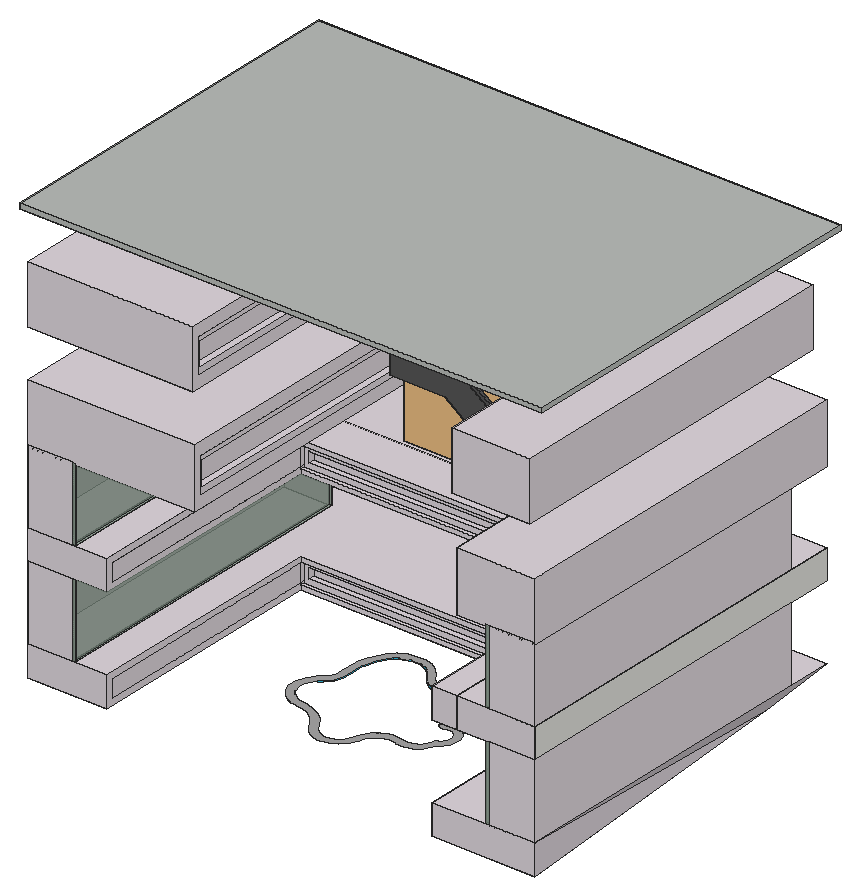
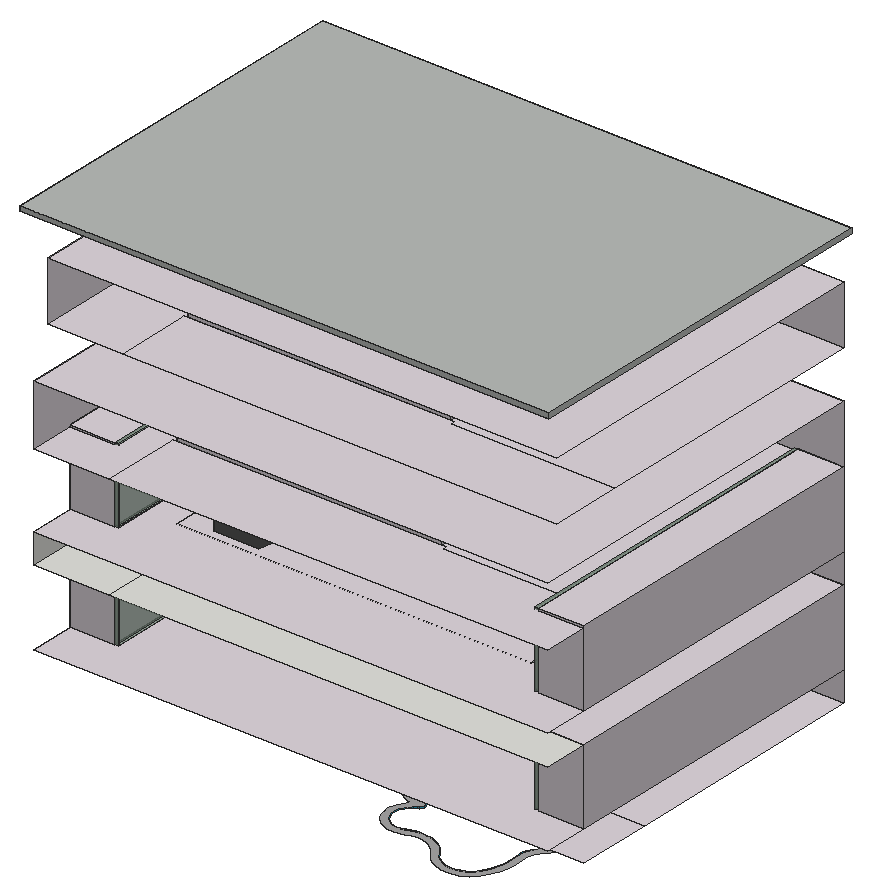
# SketchUp Ruby script. Lengths in inches.
U = 1.inch
M = Sketchup.active_model
def pt(a) = Geom::Point3d.new(a.map { |v| v * U })
def face(e, loops, mat)
  f = e.add_face(loops[0].map { |a| pt(a) })
  loops[1..].each { |l| e.add_face(l.map { |a| pt(a) }).erase! }
  f.material = f.back_material = mat if mat
  f
end
# faces: each face lists its corners as indices into pts; further lists are holes
def faces(e, pts, list, mat = nil) = list.each { |f| face(e, (f[0].is_a?(Array) ? f : [f]).map { |l| l.map { |i| pts[i] } }, mat) }
# xy, xz, yz: faces in a plane at the given z, y or x. An outline is a flat list of corners, or four numbers for a rectangle; further outlines are holes
def ring(l) = l.size == 4 ? [[l[0], l[1]], [l[2], l[1]], [l[2], l[3]], [l[0], l[3]]] : l.each_slice(2).to_a
def flat(e, list, mat, &to3) = list.each { |f| face(e, (f[0].is_a?(Array) ? f : [f]).map { |l| ring(l).map { |u, v| to3.(u, v) } }, mat) }
def xy(e, z, list, mat = nil) = flat(e, list, mat) { |x, y| [x, y, z] }
def xz(e, y, list, mat = nil) = flat(e, list, mat) { |x, z| [x, y, z] }
def yz(e, x, list, mat = nil) = flat(e, list, mat) { |y, z| [x, y, z] }
def lines(e, pts, list) = list.each { |a, b| e.add_line(pt(pts[a]), pt(pts[b])) }
# prism: a flat outline (further loops are holes) pulled along v
def prism(e, loops, v, mat = nil)
  f = face(e, loops, mat); d = Geom::Vector3d.new(v.map { |x| x * U })
  f.pushpull(f.normal.samedirection?(d) ? d.length : -d.length)
end
def box(e, o, s, mat = nil) = prism(e, [[o, [o[0] + s[0], o[1], o[2]], [o[0] + s[0], o[1] + s[1], o[2]], [o[0], o[1] + s[1], o[2]]]], [0, 0, s[2]], mat)
def at(x, y, z, deg = 0) = Geom::Transformation.translation(pt([x, y, z])) * Geom::Transformation.rotation(ORIGIN, Z_AXIS, deg.degrees)
def axes(o, x, y, z) = Geom::Transformation.new([*x, 0, *y, 0, *z, 0, *pt(o).to_a, 1])
def part(name) = M.definitions.add(name)
# library, detail: a bought-in or finely detailed component or shape, given as its bounding box
def library(name, o, s) = part(name).tap { |d| box(d.entities, o, s) }
def detail(e, o, s) = box(e.add_group.entities, o, s)
def put(e, d, t, mat = nil) = e.add_instance(d, t).tap { |i| i.material = mat if mat }
def group(e, t, mat = nil) = e.add_group.tap { |g| g.transformation = t; g.material = mat if mat }.entities
root = M.entities
M.materials.add("0265 AP 7147 LAVENDER LAUGH").color = [222, 214, 220]
M.materials.add("Epoch Sky_ Double Herringbone (VR1MIV)").color = [184, 188, 184]
M.materials.add("[Color M06]").color = [86, 86, 86]
M.materials.add("[Stone_Granite_Midnite]").color = [209, 202, 204]
M.materials.add("[Stone_Vein_Gray]").color = [166, 165, 165]
M.materials.add("[Translucent Glass Corrugated]").color = [141, 158, 145]
M.materials["[Translucent Glass Corrugated]"].alpha = 0.8
M.materials.add("[Water Sparkling]").color = [45, 182, 216]
c1 = part("Group\#8")
xy(c1.entities,0,[[0,0,0,395.68,120,395.68,120,389.68,127.1,389.68,127.1,0],[650.35,0,650.35,389.68,656.35,389.68,656.35,515.68,776.35,515.68,816,0],[120,389.68,120,395.68,0,395.68,0,515.68,656.35,515.68,656.35,389.68]])
xy(c1.entities,5.68,[[650.35,5.68,659.41,456.32]])
xy(c1.entities,7.1,[[127.1,389.68,649.25,396.37]])
xy(c1.entities,9.43,[[126,9.43,127.1,452.57]])
xy(c1.entities,11.36,[[659.41,11.36,671.48,450.64]])
xy(c1.entities,14.05,[[114.8125,14.05,126,447.95]])
xy(c1.entities,15.33,[[135.33,396.37,641.02,406.43]])
xy(c1.entities,32.67,[[135.33,396.37,641.02,406.43]])
xy(c1.entities,33.95,[[114.8125,14.05,126,447.95]])
xy(c1.entities,36.64,[[659.41,11.36,671.48,450.64]])
xy(c1.entities,38.57,[[126,9.43,127.1,452.57]])
xy(c1.entities,40.9,[[127.1,389.68,649.25,396.37]])
xy(c1.entities,42.32,[[650.35,5.68,659.41,456.32]])
xy(c1.entities,48,[[0,0,127.1,0,127.1,389.68,650.35,389.68,650.35,0,816,0,816,588,0,588]])
xz(c1.entities,0,[[0,0,127.1,48],[650.35,0,816,48]])
xz(c1.entities,5.68,[[650.35,5.68,659.41,42.32]])
xz(c1.entities,9.43,[[126,9.43,127.1,38.57]])
xz(c1.entities,11.36,[[659.41,11.36,671.48,36.64]])
xz(c1.entities,14.05,[[114.8125,14.05,126,33.95]])
xz(c1.entities,389.68,[[127.1,0,650.35,0,650.35,48,127.1,48,127.1,40.9,649.25,40.9,649.25,7.1,127.1,7.1]])
xz(c1.entities,396.37,[[[127.1,7.1,649.25,40.9],[135.33,15.33,641.02,32.67]]])
xz(c1.entities,406.43,[[135.33,15.33,641.02,32.67]])
xz(c1.entities,447.95,[[114.8125,14.05,126,33.95]])
xz(c1.entities,450.64,[[659.41,11.36,671.48,36.64]])
xz(c1.entities,452.57,[[126,9.43,127.1,38.57]])
xz(c1.entities,456.32,[[650.35,5.68,659.41,42.32]])
yz(c1.entities,114.8125,[[14.05,14.05,447.95,33.95]])
yz(c1.entities,126,[[[9.43,9.43,452.57,38.57],[14.05,14.05,447.95,33.95]]])
yz(c1.entities,127.1,[[0,0,389.68,0,389.68,9.43,9.43,9.43,9.43,38.57,389.68,38.57,389.68,48,0,48],[389.68,7.1,396.37,9.43],[9.43,9.43,389.68,38.57],[389.68,9.43,396.37,38.57],[389.68,38.57,396.37,40.9]])
yz(c1.entities,135.33,[[396.37,15.33,406.43,32.67]])
yz(c1.entities,641.02,[[396.37,15.33,406.43,32.67]])
yz(c1.entities,649.25,[[389.68,7.1,396.37,40.9]])
yz(c1.entities,650.35,[[0,0,0,48,389.68,48,389.68,42.32,5.68,42.32,5.68,5.68,389.68,5.68,389.68,0],[5.68,5.68,389.68,42.32]])
yz(c1.entities,659.41,[[[5.68,5.68,456.32,42.32],[11.36,11.36,450.64,36.64]]])
yz(c1.entities,671.48,[[11.36,11.36,450.64,36.64]])
p = [[816,0,0],[776.35,515.68,0],[816,0,48],[816,588,48]]
faces(c1.entities,p,[[0,1,2],[3,2,1]])
c2 = part("Group41\#1")
p = [[514.8125,1.1875,0],[1.1875,1.1875,0],[1.1875,118.8125,0],[514.8125,118.8125,0]]
lines(c2.entities,p,[[0,1],[1,2],[2,3],[3,0]])
c3 = part("Group42\#1")
xy(c3.entities,2.9375,[[1.1875,1.1875,514.8125,118.8125]])
c4 = part("Group40\#1")
prism(c4.entities,[[[516,120,0],[516,0,0],[0,0,0],[0,120,0]],[[1.1875,118.8125,0],[1.1875,1.1875,0],[514.8125,1.1875,0],[514.8125,118.8125,0]]],[0,0,5.875])
put(c4.entities,c2,at(0,0,0))
put(c4.entities,c3,at(0,0,0))
c5 = part("Group\#11")
xy(c5.entities,0,[[0,72,72,588]])
xy(c5.entities,120,[[0,72,72,588]])
xz(c5.entities,72,[[0,0,72,120]])
xz(c5.entities,588,[[0,0,72,120]])
yz(c5.entities,0,[[72,0,588,120]])
put(c5.entities,c4,axes([72,72,0],[0,1,0],[0,0,1],[1,0,0]),"[Translucent Glass Corrugated]")
c6 = library("Group9\#2",[-51.57,-27.17,6.46],[325.75,3.15,149.29])
c7 = part("Group8\#1")
prism(c7.entities,[[[-38.42,-26,8.24],[-37.21,-26,8.08],[-35.98,-26,8.03],[-35.98,-26,14.02],[-0.59,-26,14.02],[3.6,-26,14.2],[7.75,-26,14.75],[11.84,-26,15.65],[15.84,-26,16.91],[19.71,-26,18.52],[23.43,-26,20.45],[211.27,-26,128.91],[213.125,-26,129.875],[215.06,-26,130.68],[217.06,-26,131.31],[219.1,-26,131.76],[221.18,-26,132.03],[223.27,-26,132.125],[258.59,-26,132.125],[258.59,-26,126.14],[259.81,-26,126.2],[261.02,-26,126.35],[262.22,-26,126.62],[263.38,-26,126.99],[264.51,-26,127.45],[265.6,-26,128.02],[266.63,-26,128.68],[267.6,-26,129.42],[268.5,-26,130.25],[269.33,-26,131.15],[270.07,-26,132.12],[270.73,-26,133.15],[271.29,-26,134.23],[271.76,-26,135.36],[272.125,-26,136.53],[272.39,-26,137.72],[272.55,-26,138.9375],[272.6,-26,140.16],[272.55,-26,141.38],[272.39,-26,142.59],[272.125,-26,143.79],[271.76,-26,144.95],[271.29,-26,146.08],[270.73,-26,147.17],[270.07,-26,148.2],[269.33,-26,149.17],[268.5,-26,150.07],[267.6,-26,150.89],[266.63,-26,151.64],[265.6,-26,152.3],[264.51,-26,152.86],[263.38,-26,153.33],[262.22,-26,153.7],[261.02,-26,153.96],[259.81,-26,154.12],[258.59,-26,154.17],[223.27,-26,154.17],[219.26,-26,154],[215.27,-26,153.47],[211.35,-26,152.6],[207.52,-26,151.4],[203.81,-26,149.86],[200.24,-26,148],[12.4,-26,39.54],[10.39,-26,38.5],[8.3,-26,37.63],[6.13,-26,36.95],[3.92,-26,36.46],[1.67,-26,36.16],[-0.59,-26,36.0625],[-35.98,-26,36.0625],[-37.21,-26,36.01],[-38.42,-26,35.85],[-39.61,-26,35.59],[-40.78,-26,35.22],[-41.91,-26,34.75],[-42.99,-26,34.19],[-44.02,-26,33.53],[-44.99,-26,32.78],[-45.89,-26,31.96],[-46.72,-26,31.06],[-47.47,-26,30.09],[-48.12,-26,29.06],[-48.6875,-26,27.97],[-49.15,-26,26.84],[-49.52,-26,25.67],[-49.79,-26,24.48],[-49.95,-26,23.27],[-50,-26,22.05],[-49.95,-26,20.83],[-49.79,-26,19.61],[-49.52,-26,18.42],[-49.15,-26,17.25],[-48.6875,-26,16.125],[-48.12,-26,15.04],[-47.47,-26,14.01],[-46.72,-26,13.04],[-45.89,-26,12.14],[-44.99,-26,11.3125],[-44.02,-26,10.57],[-42.99,-26,9.91],[-41.91,-26,9.34],[-40.78,-26,8.875],[-39.61,-26,8.51]]],[0,0.8125,0])
c8 = part("Group7\#1")
prism(c8.entities,[[[-35.98,-31.5,14.02],[-35.98,-31.5,0],[0,-31.5,0],[204.57,-31.5,118.11],[258.59,-31.5,118.11],[258.59,-31.5,132.125],[223.27,-31.5,132.125],[222.02,-31.5,132.09],[220.76,-31.5,131.99],[219.52,-31.5,131.83],[218.28,-31.5,131.6],[217.06,-31.5,131.31],[215.85,-31.5,130.95],[214.67,-31.5,130.53],[213.51,-31.5,130.05],[212.37,-31.5,129.51],[211.27,-31.5,128.91],[23.41,-31.5,20.45],[21.2,-31.5,19.25],[18.93,-31.5,18.16],[16.61,-31.5,17.2],[14.24,-31.5,16.36],[11.83,-31.5,15.65],[9.39,-31.5,15.0625],[6.92,-31.5,14.61],[4.43,-31.5,14.28],[1.92,-31.5,14.08],[-0.59,-31.5,14.02]]],[0,11.8125,0])
c9 = part("Group8\#2")
prism(c9.entities,[[[-38.42,-26,8.24],[-37.21,-26,8.08],[-35.98,-26,8.03],[-35.98,-26,14.02],[-0.59,-26,14.02],[3.6,-26,14.2],[7.75,-26,14.75],[11.84,-26,15.65],[15.84,-26,16.91],[19.71,-26,18.52],[23.43,-26,20.45],[211.27,-26,128.91],[213.125,-26,129.875],[215.06,-26,130.68],[217.06,-26,131.31],[219.1,-26,131.76],[221.18,-26,132.03],[223.27,-26,132.125],[258.59,-26,132.125],[258.59,-26,126.14],[259.81,-26,126.2],[261.02,-26,126.35],[262.22,-26,126.62],[263.38,-26,126.99],[264.51,-26,127.45],[265.6,-26,128.02],[266.63,-26,128.68],[267.6,-26,129.42],[268.5,-26,130.25],[269.33,-26,131.15],[270.07,-26,132.12],[270.73,-26,133.15],[271.29,-26,134.23],[271.76,-26,135.36],[272.125,-26,136.53],[272.39,-26,137.72],[272.55,-26,138.9375],[272.6,-26,140.16],[272.55,-26,141.38],[272.39,-26,142.59],[272.125,-26,143.79],[271.76,-26,144.95],[271.29,-26,146.08],[270.73,-26,147.17],[270.07,-26,148.2],[269.33,-26,149.17],[268.5,-26,150.07],[267.6,-26,150.89],[266.63,-26,151.64],[265.6,-26,152.3],[264.51,-26,152.86],[263.38,-26,153.33],[262.22,-26,153.7],[261.02,-26,153.96],[259.81,-26,154.12],[258.59,-26,154.17],[223.27,-26,154.17],[219.26,-26,154],[215.27,-26,153.47],[211.35,-26,152.6],[207.52,-26,151.4],[203.81,-26,149.86],[200.24,-26,148],[12.4,-26,39.54],[10.39,-26,38.5],[8.3,-26,37.63],[6.13,-26,36.95],[3.92,-26,36.46],[1.67,-26,36.16],[-0.59,-26,36.0625],[-35.98,-26,36.0625],[-37.21,-26,36.01],[-38.42,-26,35.85],[-39.61,-26,35.59],[-40.78,-26,35.22],[-41.91,-26,34.75],[-42.99,-26,34.19],[-44.02,-26,33.53],[-44.99,-26,32.78],[-45.89,-26,31.96],[-46.72,-26,31.06],[-47.47,-26,30.09],[-48.12,-26,29.06],[-48.6875,-26,27.97],[-49.15,-26,26.84],[-49.52,-26,25.67],[-49.79,-26,24.48],[-49.95,-26,23.27],[-50,-26,22.05],[-49.95,-26,20.83],[-49.79,-26,19.61],[-49.52,-26,18.42],[-49.15,-26,17.25],[-48.6875,-26,16.125],[-48.12,-26,15.04],[-47.47,-26,14.01],[-46.72,-26,13.04],[-45.89,-26,12.14],[-44.99,-26,11.3125],[-44.02,-26,10.57],[-42.99,-26,9.91],[-41.91,-26,9.34],[-40.78,-26,8.875],[-39.61,-26,8.51]]],[0,0.8125,0])
c10 = part("Group\#7")
put(c10.entities,c6,axes([389.09,-25,81.45],[-1.32087,0,0],[0,-1.27,0],[0,0,1.97633]))
g1 = group(c10.entities,at(0,0,0))
put(g1,c7,axes([389.09,40,90.88],[-1.32087,0,0],[0,-1.27,0],[0,0,1.97633]))
put(g1,c8,axes([389.09,40,90.88],[-1.32087,0,0],[0,-1.27,0],[0,0,1.97633]))
put(g1,c9,axes([389.09,-25,90.88],[-1.32087,0,0],[0,-1.27,0],[0,0,1.97633]))
g2 = group(g1,at(0,0,0))
xy(g2,0,[[389.09,0,484.2,80.01]])
xy(g2,48.01,[[436.62,0,484.2,80.01]])
xy(g2,62.63,[[422.02,15,436.62,65.01]])
xy(g2,74.76,[[399.75,15,422.02,65.01]])
xy(g2,83.13,[[377.47,15,399.75,65.01]])
xy(g2,90.88,[[389.09,0,436.62,15],[389.09,65.01,436.62,80.01]])
xy(g2,100.22,[[356.01,15,378.28,65.01]])
xy(g2,118.11,[[335.29,15,357.57,65.01]])
xy(g2,118.58,[[389.87,0,436.62,15]])
xy(g2,136.01,[[314.57,15,336.85,65.01]])
xy(g2,153.9,[[293.86,15,316.13,65.01]])
xy(g2,171.8,[[273.14,15,295.42,65.01]])
xy(g2,189.7,[[252.42,15,274.7,65.01]])
xy(g2,207.59,[[231.71,15,253.98,65.01]])
xy(g2,225.49,[[210.99,15,233.27,65.01]])
xy(g2,233.42,[[0,0,118.88,80.01]])
xy(g2,243.38,[[190.28,15,212.55,65.01]])
xy(g2,261.28,[[169.56,15,191.84,65.01]])
xy(g2,279.18,[[148.84,15,171.12,65.01]])
xy(g2,297.07,[[128.125,15,150.4,65.01]])
xy(g2,314.97,[[107.41,15,129.6875,65.01]])
xy(g2,324.3,[[0,0,47.53,0,47.53,65.01,118.88,65.01,118.88,80.01,0,80.01],[47.53,0,118.88,15],[47.53,15,63.67,65.01],[63.67,15,85.95,65.01],[85.95,15,108.22,65.01]])
xy(g2,352,[[47.53,0,94.18,15]])
xz(g2,0,[[389.09,0,484.2,0,484.2,48.01,436.62,48.01,436.62,90.88,389.09,90.88,118.88,324.3,0,324.3,0,233.42,118.88,233.42],[389.09,90.88,436.62,90.88,436.62,118.58,389.87,118.58,386.55,118.71,383.25,119.1,379.95,119.75,376.69,120.65,373.46,121.8125,370.28,123.22,367.15,124.88,364.09,126.78,361.09,128.92,358.18,131.29,110.04,345.65,108.58,346.83,107.08,347.9,105.54,348.85,103.98,349.68,102.39,350.39,100.77,350.97,99.14,351.42,97.49,351.74,95.84,351.9375,94.18,352,47.53,352,47.53,324.3,118.88,324.3]])
xz(g2,15,[[422.02,62.63,436.62,90.88],[399.75,74.76,422.02,90.88],[377.47,83.13,389.09,90.88],[389.09,83.13,399.75,90.88],[389.09,90.88,378.28,100.22,357.57,118.11,336.85,136.01,316.13,153.9,295.42,171.8,274.7,189.7,253.98,207.59,233.27,225.49,212.55,243.38,191.84,261.28,171.12,279.18,150.4,297.07,129.6875,314.97,118.88,324.3,47.53,324.3,47.53,352,94.18,352,95.84,351.9375,97.49,351.74,99.14,351.42,100.77,350.97,102.39,350.39,103.98,349.68,105.54,348.85,107.08,347.9,108.58,346.83,110.04,345.65,358.18,131.29,361.09,128.92,364.09,126.78,367.15,124.88,370.28,123.22,373.46,121.8125,376.69,120.65,379.95,119.75,383.25,119.1,386.55,118.71,389.87,118.58,436.62,118.58,436.62,90.88]])
xz(g2,65.01,[[422.02,62.63,436.62,90.88],[399.75,74.76,422.02,90.88],[377.47,83.13,389.09,90.88],[389.09,83.13,399.75,90.88]])
xz(g2,80.01,[[389.09,0,118.88,233.42,0,233.42,0,324.3,118.88,324.3,389.09,90.88,436.62,90.88,436.62,48.01,484.2,48.01,484.2,0]])
yz(g2,0,[[0,233.42,80.01,324.3]])
yz(g2,47.53,[[0,324.3,15,352]])
yz(g2,377.47,[[15,83.13,65.01,90.88]])
yz(g2,399.75,[[15,74.76,65.01,83.13]])
yz(g2,422.02,[[15,62.63,65.01,74.76]])
yz(g2,436.62,[[0,48.01,15,90.88],[15,48.01,65.01,62.63],[65.01,48.01,80.01,90.88],[0,90.88,15,118.58]])
yz(g2,484.2,[[0,0,80.01,48.01]])
p = [[389.09,80.01,0],[389.09,0,0],[118.88,0,233.42],[118.88,80.01,233.42],[378.28,15,100.22],[389.09,15,90.88],
  [389.09,0,90.88],[118.88,0,324.3],[118.88,15,324.3],[129.6875,15,314.97],[150.4,15,297.07],[171.12,15,279.18],
  [191.84,15,261.28],[212.55,15,243.38],[233.27,15,225.49],[253.98,15,207.59],[274.7,15,189.7],[295.42,15,171.8],
  [316.13,15,153.9],[336.85,15,136.01],[357.57,15,118.11],[378.28,65.01,100.22],[377.47,15,90.88],[377.47,65.01,90.88],
  [357.57,65.01,118.11],[356.01,15,100.22],[356.01,65.01,100.22],[336.85,65.01,136.01],[335.29,15,118.11],[335.29,65.01,118.11],
  [389.87,15,118.58],[386.55,15,118.71],[386.55,0,118.71],[389.87,0,118.58],[383.25,15,119.1],[383.25,0,119.1],
  [379.95,15,119.75],[379.95,0,119.75],[376.69,15,120.65],[376.69,0,120.65],[373.46,15,121.8125],[373.46,0,121.8125],
  [370.28,15,123.22],[370.28,0,123.22],[367.15,15,124.88],[367.15,0,124.88],[364.09,15,126.78],[364.09,0,126.78],
  [361.09,15,128.92],[361.09,0,128.92],[358.18,15,131.29],[358.18,0,131.29],[110.04,15,345.65],[110.04,0,345.65],
  [316.13,65.01,153.9],[314.57,15,136.01],[314.57,65.01,136.01],[295.42,65.01,171.8],[293.86,15,153.9],[293.86,65.01,153.9],
  [274.7,65.01,189.7],[273.14,15,171.8],[273.14,65.01,171.8],[253.98,65.01,207.59],[252.42,15,189.7],[252.42,65.01,189.7],
  [233.27,65.01,225.49],[231.71,15,207.59],[231.71,65.01,207.59],[212.55,65.01,243.38],[210.99,15,225.49],[210.99,65.01,225.49],
  [191.84,65.01,261.28],[190.28,15,243.38],[190.28,65.01,243.38],[171.12,65.01,279.18],[169.56,15,261.28],[169.56,65.01,261.28],
  [150.4,65.01,297.07],[148.84,15,279.18],[148.84,65.01,279.18],[129.6875,65.01,314.97],[128.125,15,297.07],[128.125,65.01,297.07],
  [108.22,65.01,324.3],[108.22,15,324.3],[107.41,15,314.97],[107.41,65.01,314.97],[108.58,15,346.83],[108.58,0,346.83],
  [107.08,15,347.9],[107.08,0,347.9],[105.54,15,348.85],[105.54,0,348.85],[103.98,15,349.68],[103.98,0,349.68],
  [102.39,15,350.39],[102.39,0,350.39],[100.77,15,350.97],[100.77,0,350.97],[99.14,15,351.42],[99.14,0,351.42],
  [97.49,15,351.74],[97.49,0,351.74],[95.84,15,351.9375],[95.84,0,351.9375],[94.18,15,352],[94.18,0,352]]
faces(g2,p,[[0,1,2,3],[4,5,6,7,8,9,10,11,12,13,14,15,16,17,18,19,20],[21,4,22,23],[24,20,25,26],[27,19,28,29],[30,31,32,33],[31,34,35,32],[34,36,37,35],
  [36,38,39,37],[38,40,41,39],[40,42,43,41],[42,44,45,43],[44,46,47,45],[46,48,49,47],[48,50,51,49],[50,52,53,51],
  [54,18,55,56],[57,17,58,59],[60,16,61,62],[63,15,64,65],[66,14,67,68],[69,13,70,71],[72,12,73,74],[75,11,76,77],
  [78,10,79,80],[81,9,82,83],[84,85,86,87],[52,88,89,53],[88,90,91,89],[90,92,93,91],[92,94,95,93],[94,96,97,95],
  [96,98,99,97],[98,100,101,99],[100,102,103,101],[102,104,105,103],[104,106,107,105]])
c11 = part("Group\#4")
xy(c11.entities,0,[[0,0,0,468,261.34,468,261.34,462,268.44,462,268.44,0],[690,0,690,462,696,462,696,588,816,588,816,0],[261.34,462,261.34,468,0,468,0,588,696,588,696,462]])
xy(c11.entities,5.68,[[690,5.68,699.0625,456.32]])
xy(c11.entities,7.1,[[268.44,462,688.9,468.6875]])
xy(c11.entities,9.43,[[267.34,9.43,268.44,452.57]])
xy(c11.entities,11.36,[[699.0625,11.36,711.125,450.64]])
xy(c11.entities,14.05,[[256.15,14.05,267.34,447.95]])
xy(c11.entities,15.33,[[276.67,468.6875,680.67,478.75]])
xy(c11.entities,32.67,[[276.67,468.6875,680.67,478.75]])
xy(c11.entities,33.95,[[256.15,14.05,267.34,447.95]])
xy(c11.entities,36.64,[[699.0625,11.36,711.125,450.64]])
xy(c11.entities,38.57,[[267.34,9.43,268.44,452.57]])
xy(c11.entities,40.9,[[268.44,462,688.9,468.6875]])
xy(c11.entities,42.32,[[690,5.68,699.0625,456.32]])
xy(c11.entities,48,[[0,0,268.44,0,268.44,462,690,462,690,0,816,0,816,588,0,588]])
xz(c11.entities,0,[[0,0,268.44,48],[690,0,816,48]])
xz(c11.entities,5.68,[[690,5.68,699.0625,42.32]])
xz(c11.entities,9.43,[[267.34,9.43,268.44,38.57]])
xz(c11.entities,11.36,[[699.0625,11.36,711.125,36.64]])
xz(c11.entities,14.05,[[256.15,14.05,267.34,33.95]])
xz(c11.entities,447.95,[[256.15,14.05,267.34,33.95]])
xz(c11.entities,450.64,[[699.0625,11.36,711.125,36.64]])
xz(c11.entities,452.57,[[267.34,9.43,268.44,38.57]])
xz(c11.entities,456.32,[[690,5.68,699.0625,42.32]])
xz(c11.entities,462,[[268.44,0,690,0,690,48,268.44,48,268.44,40.9,688.9,40.9,688.9,7.1,268.44,7.1]])
xz(c11.entities,468.6875,[[[268.44,7.1,688.9,40.9],[276.67,15.33,680.67,32.67]]])
xz(c11.entities,478.75,[[276.67,15.33,680.67,32.67]])
yz(c11.entities,256.15,[[14.05,14.05,447.95,33.95]])
yz(c11.entities,267.34,[[[9.43,9.43,452.57,38.57],[14.05,14.05,447.95,33.95]]])
yz(c11.entities,268.44,[[[0,0,462,48],[9.43,9.43,452.57,38.57]],[462,7.1,468.6875,40.9]])
yz(c11.entities,276.67,[[468.6875,15.33,478.75,32.67]])
yz(c11.entities,680.67,[[468.6875,15.33,478.75,32.67]])
yz(c11.entities,688.9,[[462,7.1,468.6875,40.9]])
yz(c11.entities,690,[[[0,0,462,48],[5.68,5.68,456.32,42.32]]])
yz(c11.entities,699.0625,[[[5.68,5.68,456.32,42.32],[11.36,11.36,450.64,36.64]]])
yz(c11.entities,711.125,[[11.36,11.36,450.64,36.64]])
yz(c11.entities,816,[[0,0,588,48]])
c12 = part("Group\#1")
box(c12.entities,[0,0,0],[840,600,8])
xy(root,22.57,[[190.8,304.2,185,306.78,190.22,304.25],[182.64,323.65,179.63,327.58,181.13,325.16],[179.63,327.58,178.33,329.6875,178.77,328.71],[404.72,421.12,404.22,423.78,403.55,426.41]],"[Stone_Granite_Midnite]")
xy(root,22.57,[[[283.33,249.2,295.21,251.08,306.59,257.15,316.71,268.8125,321.12,280.93,323.65,288.67,326.86,293.88,336.05,301.87,343.61,304.89,349.66,305.77,357.77,305.03,361.3125,304.09,361.46,304.05,361.75,303.98,362.12,303.88,374.31,303.22,386.02,306.66,397.57,315.62,403.8,326.12,405.24,330.8,408.45,332.9,412.68,336.8,417.72,344.9,419.35,350.41,419.2,361.84,417.85,365.55,416.58,369.03,412.05,374.99,411.92,375.15,411.5,375.7,411.39,375.86,408,378.45,406.49,379.59,404.5625,381.0625,397.375,383.69,391.67,384.34,395.43,388.24,402.35,399.82,404.78,409.65,405.01,411.67,405.16,413.01,405.11,413.92,405.01,415.75,404.875,418.25,404.85,418.74,404.72,421.12,403.55,426.41,401.69,431.49,397.7,438.5625,388.23,448.17,376.17,454.21,373.55,454.92,372.22,455.19,370.9,455.46,365.51,456.01,361.45,455.94,356.08,455.24,352.13,454.28,347.06,452.38,343.04,450.82,338.89,449.63,336.07,449.08,321.75,449.2,310.82,452.68,299.07,460.86,290.2,472.77,281.15,482.86,277.1,485.93,272.78,488.64,269.76,490.17,256.83,494.2,243.29,494.66,230.125,491.51,218.26,484.97,208.5625,475.52,201.7,464.27,196.78,452.45,193.5,440.07,191.92,427.37,192.56,412.99,193.05,402.18,192.09,396.23,190.37,391.69,186.71,385.52,176.48,376.24,167.83,364.6875,163.43,350.94,163.75,336.51,167.41,325.53,175.8,313.79,185,306.78,190.8,304.2,192.9375,303.25,195.08,302.62,198.55,301.8,204.3,301.11,211.11,300.28,224.0625,295.92,235.37,288.23,244.19,277.79,249.93,267.22,256.55,259.29,262.77,254.64,269.78,251.32,277.3125,249.46],[285.14,260.64,279.6875,260.875,272.69,262.85,263.78,269.07,256.8,280.34,246.85,293.88,237.2,302,222.15,309.47,207.75,312.44,195.29,314.93,185.875,321.17,184.68,321.95,183.38,323.65,180.37,327.58,179.51,328.71,179.07,329.6875,176.89,334.54,175.3,342.9,175.58,349.29,177.12,355.49,179.32,359.76,180.53,362.1,182.23,364.22,185.18,367.91,190.66,372.36,199.66,382.97,204.6,395.97,204.93,409.88,204.16,426.72,204.67,432.32,205.55,437.88,210.42,454.01,216.84,466.29,221.88,472.31,228.02,477.2,232.61,479.72,239.94,482.01,242.59,482.84,250.43,483.36,258.21,482.3125,263.21,480.75,267.96,478.54,274.42,474.08,278.17,470.42,282.8,464.08,291.74,452.62,297.28,447.88,300.27,445.8,313.41,439.59,320.48,437.85,335.01,437.24,338.62,437.7,342.2,438.39,345.72,439.32,349.18,440.48,358.06,443.74,365.78,444.49,371.35,443.56,372.94,443.3,375.26,442.59,382.09,438.92,387.73,433.6,391.81,427.01,394.03,419.58,394.39,413.77,393.09,406.125,389.86,399.08,383.44,391.84,378.01,388.36,375.49,386.45,372.99,381.41,374,375.26,379.15,370.78,380.99,370.3,384.87,371.26,386.98,372.0625,388.44,372.41,389.25,372.52,391.42,372.81,392.54,372.81,396.98,372.07,399.9375,370.6,400.11,370.52,402.01,369.57,402.8,368.82,405.28,366.47,408.67,359.41,408.79,352.69,406.89,347.41,402.51,342.3,396.5,339.28,395.4,339.02,395.35,337.39,394.54,332.57,392.01,326.58,386.78,320.36,379.82,316.19,373.49,314.65,349.9,317.29,344.3,316.67,336.1875,314.34,331.11,311.91,328.71,310.44,326.4,308.8125,322.16,305.12,318.44,300.88,311.91,288.48,307.42,274.49,303.02,268.7,297.26,264.26,292.29,262.02],[182.64,323.65,181.13,325.16,179.63,327.58,178.77,328.71,178.33,329.6875,179.63,327.58]]],"[Stone_Vein_Gray]")
p = [[190.66,372.36,22.57],[185.18,367.91,22.57],[185.18,367.91,20.71],[190.66,372.36,20.71],[199.66,382.97,22.57],[199.66,382.97,20.71],
  [374,375.26,22.57],[372.99,381.41,22.57],[372.99,381.41,20.71],[374,375.26,20.71],[375.49,386.45,22.57],[375.49,386.45,20.71],
  [204.6,395.97,22.57],[204.6,395.97,20.71],[378.01,388.36,22.57],[378.01,388.36,20.71],[383.44,391.84,22.57],[383.44,391.84,20.71],
  [389.86,399.08,22.57],[389.86,399.08,20.71],[204.93,409.88,22.57],[204.93,409.88,20.71],[393.09,406.125,22.57],[393.09,406.125,20.71],
  [394.39,413.77,22.57],[394.39,413.77,20.71],[204.16,426.72,22.57],[204.16,426.72,20.71],[394.03,419.58,22.57],[394.03,419.58,20.71],
  [391.81,427.01,22.57],[391.81,427.01,20.71],[204.67,432.32,22.57],[204.67,432.32,20.71],[387.73,433.6,22.57],[387.73,433.6,20.71],
  [205.55,437.88,22.57],[205.55,437.88,20.71],[382.09,438.92,22.57],[382.09,438.92,20.71],[335.01,437.24,22.57],[320.48,437.85,22.57],
  [320.48,437.85,20.71],[335.01,437.24,20.71],[338.62,437.7,22.57],[338.62,437.7,20.71],[342.2,438.39,22.57],[342.2,438.39,20.71],
  [313.41,439.59,22.57],[313.41,439.59,20.71],[210.42,454.01,22.57],[210.42,454.01,20.71],[345.72,439.32,22.57],[345.72,439.32,20.71],
  [375.26,442.59,22.57],[375.26,442.59,20.71],[349.18,440.48,22.57],[349.18,440.48,20.71],[300.27,445.8,22.57],[300.27,445.8,20.71],
  [358.06,443.74,22.57],[358.06,443.74,20.71],[372.94,443.3,22.57],[372.94,443.3,20.71],[371.35,443.56,22.57],[371.35,443.56,20.71],
  [365.78,444.49,22.57],[365.78,444.49,20.71],[297.28,447.88,22.57],[297.28,447.88,20.71],[291.74,452.62,22.57],[291.74,452.62,20.71],
  [282.8,464.08,22.57],[282.8,464.08,20.71],[216.84,466.29,22.57],[216.84,466.29,20.71],[278.17,470.42,22.57],[278.17,470.42,20.71],
  [221.88,472.31,22.57],[221.88,472.31,20.71],[274.42,474.08,22.57],[274.42,474.08,20.71],[228.02,477.2,22.57],[228.02,477.2,20.71],
  [267.96,478.54,22.57],[267.96,478.54,20.71],[232.61,479.72,22.57],[232.61,479.72,20.71],[263.21,480.75,22.57],[263.21,480.75,20.71],
  [239.94,482.01,22.57],[239.94,482.01,20.71],[258.21,482.3125,22.57],[258.21,482.3125,20.71],[242.59,482.84,22.57],[242.59,482.84,20.71],
  [250.43,483.36,22.57],[250.43,483.36,20.71],[319.75,437.85,22.57],[326.99,437.0625,22.57],[325.67,308.8125,22.57],[327.97,310.44,22.57]]
faces(root,p,[[0,1,2,3],[4,0,3,5],[6,7,8,9],[7,10,11,8],[12,4,5,13],[10,14,15,11],[14,16,17,15],[16,18,19,17],
  [20,12,13,21],[18,22,23,19],[22,24,25,23],[26,20,21,27],[24,28,29,25],[28,30,31,29],[32,26,27,33],[30,34,35,31],
  [36,32,33,37],[34,38,39,35],[40,41,42,43],[44,40,43,45],[46,44,45,47],[41,48,49,42],[50,36,37,51],[52,46,47,53],
  [38,54,55,39],[56,52,53,57],[48,58,59,49],[60,56,57,61],[54,62,63,55],[62,64,65,63],[64,66,67,65],[66,60,61,67],
  [58,68,69,59],[68,70,71,69],[70,72,73,71],[74,50,51,75],[72,76,77,73],[78,74,75,79],[76,80,81,77],[82,78,79,83],
  [80,84,85,81],[86,82,83,87],[84,88,89,85],[90,86,87,91],[88,92,93,89],[94,90,91,95],[92,96,97,93],[96,94,95,97]],"[Water Sparkling]")
lines(root,p,[[98,99],[100,101]])
put(root,c1,at(12,0,128),"0265 AP 7147 LAVENDER LAUGH")
put(root,c5,at(12,-72,176),"0265 AP 7147 LAVENDER LAUGH")
put(root,c5,axes([828,-72,176],[-1,0,0],[0,1,0],[0,0,1]),"0265 AP 7147 LAVENDER LAUGH")
put(root,c1,at(12,0,296),"0265 AP 7147 LAVENDER LAUGH")
g3 = group(root,at(12,0,296))
xy(g3,0,[[0,0,0,468,120,468,120,462,127.1,462,127.1,0],[690,0,690,462,696,462,696,588,816,588,816,0],[120,462,120,468,0,468,0,588,696,588,696,462]])
xy(g3,5.68,[[690,5.68,699.0625,456.32]])
xy(g3,7.1,[[127.1,462,688.9,468.6875]])
xy(g3,9.43,[[126,9.43,127.1,452.57]])
xy(g3,11.36,[[699.0625,11.36,711.125,450.64]])
xy(g3,14.05,[[114.8125,14.05,126,447.95]])
xy(g3,15.33,[[135.33,468.6875,680.67,478.75]])
xy(g3,32.67,[[135.33,468.6875,680.67,478.75]])
xy(g3,33.95,[[114.8125,14.05,126,447.95]])
xy(g3,36.64,[[699.0625,11.36,711.125,450.64]])
xy(g3,38.57,[[126,9.43,127.1,452.57]])
xy(g3,40.9,[[127.1,462,688.9,468.6875]])
xy(g3,42.32,[[690,5.68,699.0625,456.32]])
xy(g3,48,[[0,0,127.1,0,127.1,462,690,462,690,0,816,0,816,588,0,588]])
xz(g3,0,[[0,0,127.1,48],[690,0,816,48]])
xz(g3,5.68,[[690,5.68,699.0625,42.32]])
xz(g3,9.43,[[126,9.43,127.1,38.57]])
xz(g3,11.36,[[699.0625,11.36,711.125,36.64]])
xz(g3,14.05,[[114.8125,14.05,126,33.95]])
xz(g3,447.95,[[114.8125,14.05,126,33.95]])
xz(g3,450.64,[[699.0625,11.36,711.125,36.64]])
xz(g3,452.57,[[126,9.43,127.1,38.57]])
xz(g3,456.32,[[690,5.68,699.0625,42.32]])
xz(g3,462,[[127.1,0,690,0,690,48,127.1,48,127.1,40.9,688.9,40.9,688.9,7.1,127.1,7.1]])
xz(g3,468.6875,[[[127.1,7.1,688.9,40.9],[135.33,15.33,680.67,32.67]]])
xz(g3,478.75,[[135.33,15.33,680.67,32.67]])
yz(g3,114.8125,[[14.05,14.05,447.95,33.95]])
yz(g3,126,[[[9.43,9.43,452.57,38.57],[14.05,14.05,447.95,33.95]]])
yz(g3,127.1,[[[0,0,462,48],[9.43,9.43,452.57,38.57]],[462,7.1,468.6875,40.9]])
yz(g3,135.33,[[468.6875,15.33,478.75,32.67]])
yz(g3,680.67,[[468.6875,15.33,478.75,32.67]])
yz(g3,688.9,[[462,7.1,468.6875,40.9]])
yz(g3,690,[[[0,0,462,48],[5.68,5.68,456.32,42.32]]])
yz(g3,699.0625,[[[5.68,5.68,456.32,42.32],[11.36,11.36,450.64,36.64]]])
yz(g3,711.125,[[11.36,11.36,450.64,36.64]])
yz(g3,816,[[0,0,588,48]])
put(root,c5,at(12,-72,344),"0265 AP 7147 LAVENDER LAUGH")
put(root,c5,axes([828,-72,344],[-1,0,0],[0,1,0],[0,0,1]),"0265 AP 7147 LAVENDER LAUGH")
put(root,c10,axes([288.6,381.88,344],[0.7546,0,0],[0,0.82935,0],[0,0,0.64212]),"[Color M06]")
put(root,c11,axes([12.57,0,461.19],[0.99931,0,0],[0,0.99931,0],[0,0,2.00871]),"0265 AP 7147 LAVENDER LAUGH")
put(root,c10,axes([288.6,351.83,528.7],[0.84468,0,0],[0,0.82935,0],[0,0,0.64212]),"[Color M06]")
put(root,c11,axes([12,0,633.91],[0.99,0,0],[0,0.9702,0],[0,0,1.9502]),"0265 AP 7147 LAVENDER LAUGH")
put(root,c12,at(0,0,800),"Epoch Sky_ Double Herringbone (VR1MIV)")
